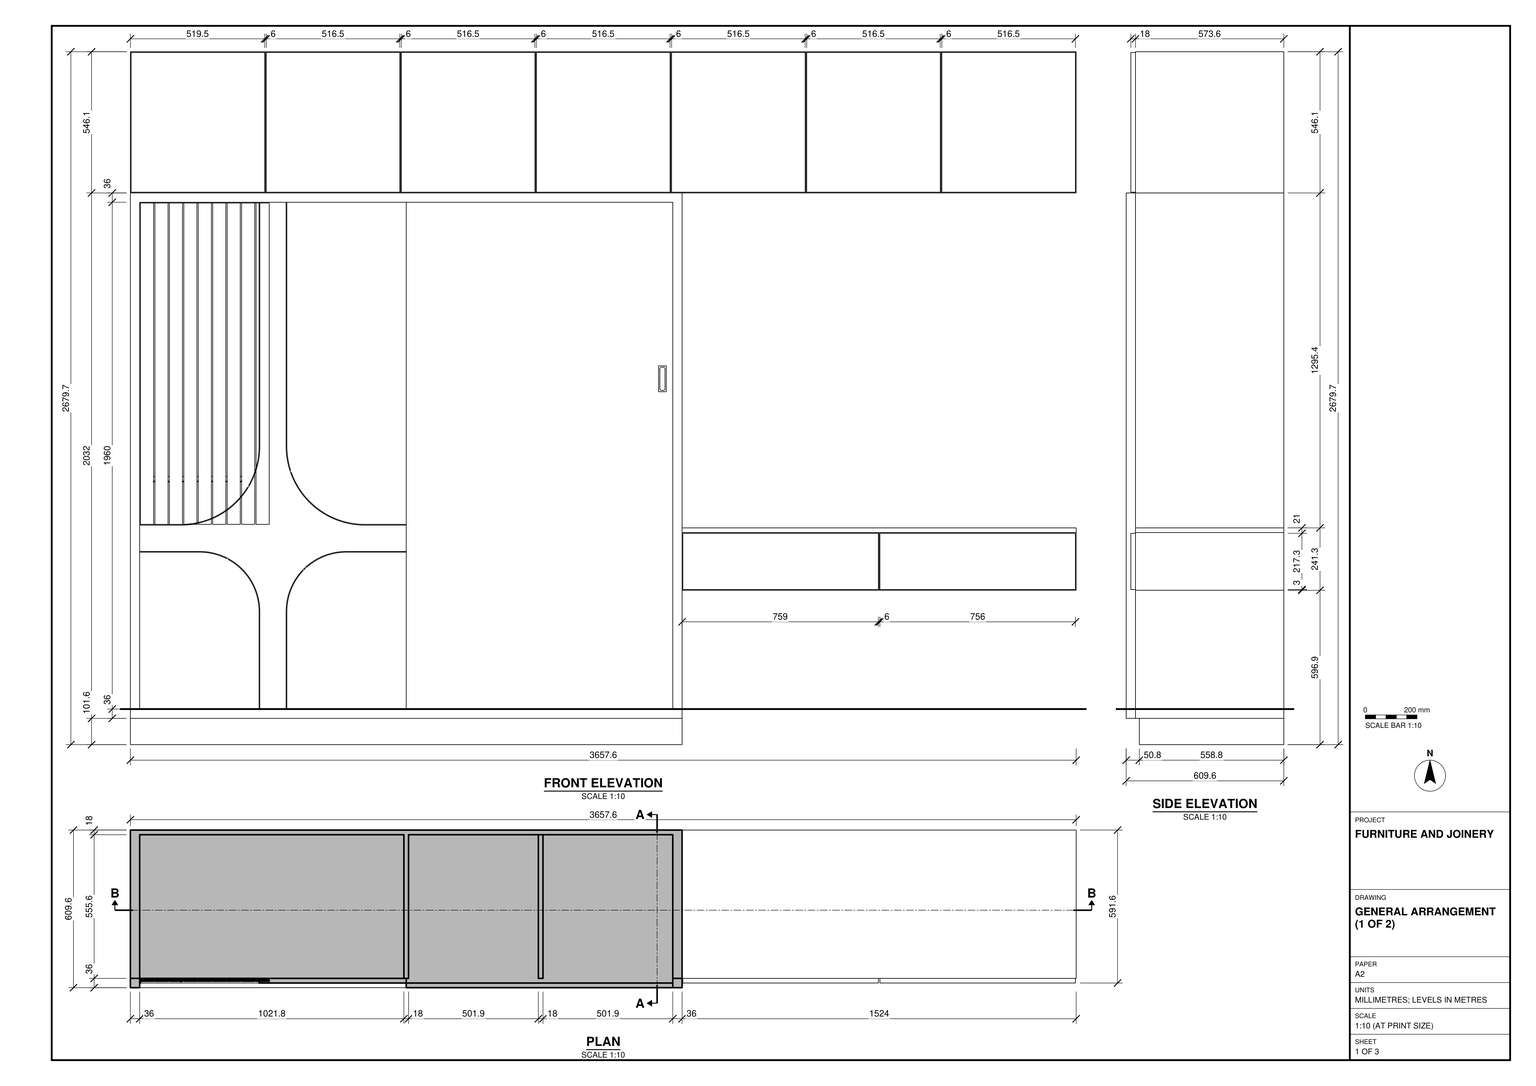
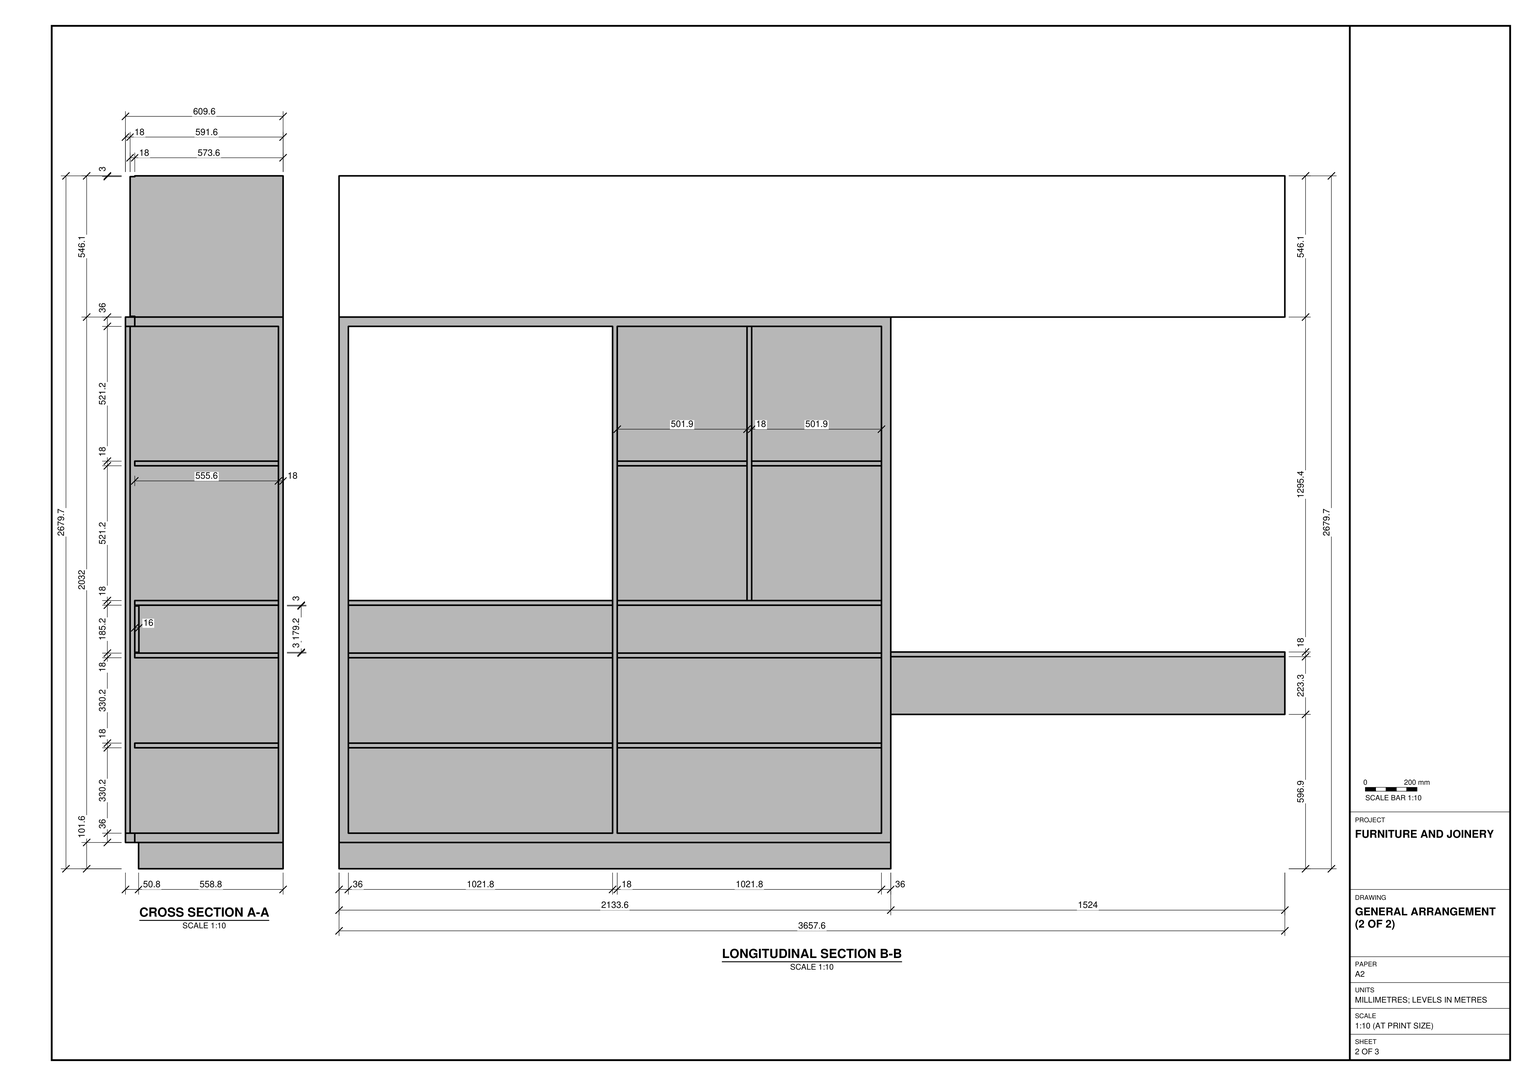
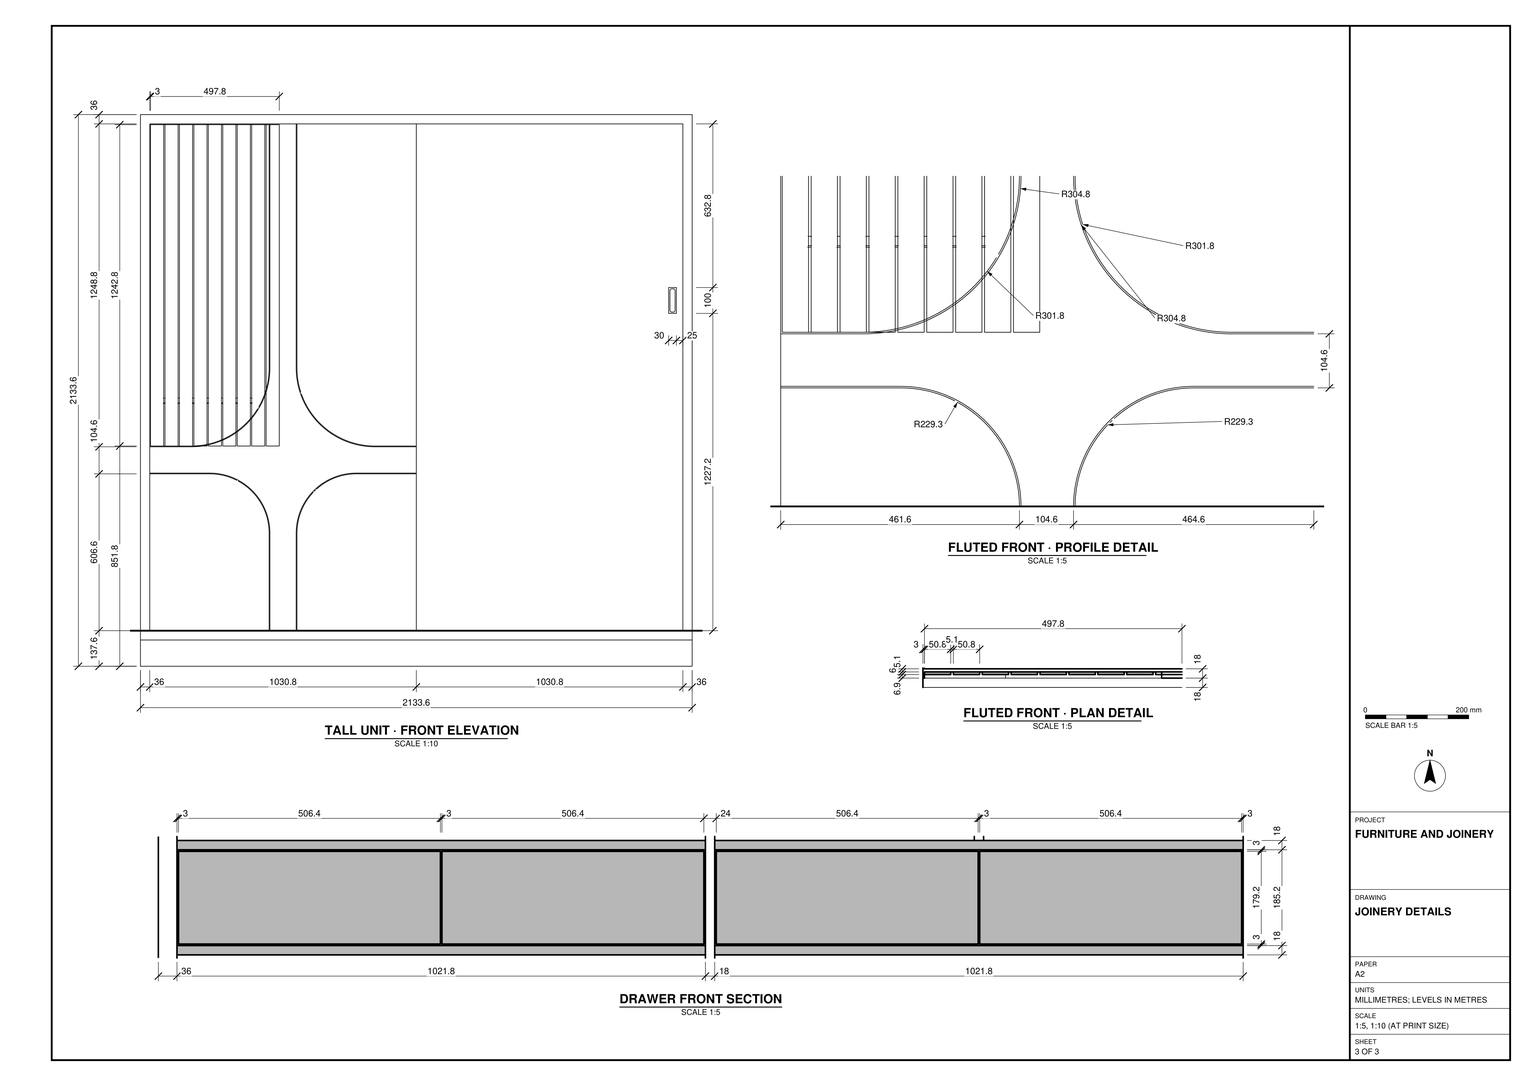
Build the storage joinery in SketchUp from task_files/diagram_01.pdf. Work in millimetres, with the underside of the plinth at ground level (±0.000, or 0 mm). Orient the front elevation along the X axis and the depth along the Y axis. The complete assembly is 3657.6 mm wide, 609.6 mm deep and 2679.7 mm high.

Run the seven overhead cupboard fronts across the full width. Below them, place the 2133.6 mm wide tall cabinet on the left and the 1524 mm wide floating drawer unit on the right. Keep the space above and below the floating unit open. Set back the tall cabinet’s plinth from its front face. Use the sections to model the cabinet interior behind the fronts, including the central partition, lower shelves, paired drawers in each bay and extra shelving in the upper right bay.

Use the third sheet for the two tall fronts. Form the vertical fluting in the upper left area of the patterned front and follow the drawn curves where the vertical and horizontal bands meet. Keep the adjoining front plain apart from its recessed rectangular pull. Model the panel thicknesses, front reveals and plinth setback shown in the sections rather than representing them with lines on a single face.

Keep the joinery units and their constituent parts separately editable as groups or components, and use components for repeated parts. Any decor or loose items may be suitable library components. Save one SketchUp model as output_files/storage_unit_with_upper_cupboards_and_floating_drawers.skp.

# SketchUp Ruby script. Lengths in millimetres.
U = 1.mm
M = Sketchup.active_model
def pt(a) = Geom::Point3d.new(a.map { |v| v * U })
def face(e, loops, mat)
  f = e.add_face(loops[0].map { |a| pt(a) })
  loops[1..].each { |l| e.add_face(l.map { |a| pt(a) }).erase! }
  f.material = f.back_material = mat if mat
  f
end
# faces: each face lists its corners as indices into pts; further lists are holes
def faces(e, pts, list, mat = nil) = list.each { |f| face(e, (f[0].is_a?(Array) ? f : [f]).map { |l| l.map { |i| pts[i] } }, mat) }
# xy, xz, yz: faces in a plane at the given z, y or x. An outline is a flat list of corners, or four numbers for a rectangle; further outlines are holes
def ring(l) = l.size == 4 ? [[l[0], l[1]], [l[2], l[1]], [l[2], l[3]], [l[0], l[3]]] : l.each_slice(2).to_a
def flat(e, list, mat, &to3) = list.each { |f| face(e, (f[0].is_a?(Array) ? f : [f]).map { |l| ring(l).map { |u, v| to3.(u, v) } }, mat) }
def xy(e, z, list, mat = nil) = flat(e, list, mat) { |x, y| [x, y, z] }
def xz(e, y, list, mat = nil) = flat(e, list, mat) { |x, z| [x, y, z] }
def yz(e, x, list, mat = nil) = flat(e, list, mat) { |y, z| [x, y, z] }
def lines(e, pts, list) = list.each { |a, b| e.add_line(pt(pts[a]), pt(pts[b])) }
# prism: a flat outline (further loops are holes) pulled along v
def prism(e, loops, v, mat = nil)
  f = face(e, loops, mat); d = Geom::Vector3d.new(v.map { |x| x * U })
  f.pushpull(f.normal.samedirection?(d) ? d.length : -d.length)
end
def box(e, o, s, mat = nil) = prism(e, [[o, [o[0] + s[0], o[1], o[2]], [o[0] + s[0], o[1] + s[1], o[2]], [o[0], o[1] + s[1], o[2]]]], [0, 0, s[2]], mat)
def at(x, y, z, deg = 0) = Geom::Transformation.translation(pt([x, y, z])) * Geom::Transformation.rotation(ORIGIN, Z_AXIS, deg.degrees)
def axes(o, x, y, z) = Geom::Transformation.new([*x, 0, *y, 0, *z, 0, *pt(o).to_a, 1])
def part(name) = M.definitions.add(name)
# library, detail: a bought-in or finely detailed component or shape, given as its bounding box
def library(name, o, s) = part(name).tap { |d| box(d.entities, o, s) }
def detail(e, o, s) = box(e.add_group.entities, o, s)
def put(e, d, t, mat = nil) = e.add_instance(d, t).tap { |i| i.material = mat if mat }
def group(e, t, mat = nil) = e.add_group.tap { |g| g.transformation = t; g.material = mat if mat }.entities
root = M.entities
c1 = part("Group\#2")
box(c1.entities,[-266.4,0,0],[1021.8,555.6,18])
c2 = part("Group\#7")
box(c2.entities,[0,0,0],[506.4,16,179.2])
c3 = part("Group\#8")
box(c3.entities,[0,0,0],[501.9,555.6,18])
xy(root,1037.2,[[1577.7,36,1595.7,591.6]])
xy(root,2097.6,[[1577.7,36,1595.7,591.6]])
xz(root,36,[[1577.7,1037.2,1595.7,2097.6]])
xz(root,591.6,[[1577.7,1037.2,1595.7,2097.6]])
yz(root,1577.7,[[36,1037.2,591.6,2097.6]])
yz(root,1595.7,[[36,1037.2,591.6,2097.6]])
p = [[1595.7,591.6,1567.4],[2097.6,591.6,1567.4]]
lines(root,p,[[0,1]])
g1 = group(root,at(0,0,101.6))
prism(g1,[[[0,36,0],[0,36,2032],[2133.6,36,2032],[2133.6,36,0]],[[2097.6,36,1996],[36,36,1996],[36,36,36],[2097.6,36,36]]],[0,-36,0])
g2 = group(root,at(0,0,0))
xy(g2,0,[[0,50.8,2133.6,609.6]])
xy(g2,101.6,[[0,36,2133.6,50.8],[0,50.8,2133.6,609.6]])
xy(g2,137.6,[[36,36,1057.8,591.6],[1075.8,36,2097.6,591.6]])
xy(g2,2097.6,[[36,36,1057.8,591.6],[1075.8,36,2097.6,591.6]])
xy(g2,2133.6,[[0,36,2133.6,609.6]])
xz(g2,36,[[[0,101.6,2133.6,2133.6],[36,137.6,2097.6,2097.6]],[1057.8,137.6,1075.8,2097.6]])
xz(g2,50.8,[[0,0,2133.6,101.6]])
xz(g2,591.6,[[36,137.6,1057.8,2097.6],[1075.8,137.6,2097.6,2097.6]])
xz(g2,609.6,[[0,0,2133.6,101.6],[0,101.6,2133.6,2133.6]])
yz(g2,0,[[50.8,0,609.6,101.6],[36,101.6,609.6,2133.6]])
yz(g2,36,[[36,137.6,591.6,2097.6]])
yz(g2,1057.8,[[36,137.6,591.6,2097.6]])
yz(g2,1075.8,[[36,137.6,591.6,2097.6]])
yz(g2,2097.6,[[36,137.6,591.6,2097.6]])
yz(g2,2133.6,[[50.8,0,609.6,101.6],[36,101.6,609.6,2133.6]])
g3 = group(root,at(36,18,137.6))
xy(g3,0,[[0,0,1030.8,18]])
xy(g3,714.2,[[3,0,159.8,12]])
xy(g3,1957,[[3,0,461.6,12]])
xy(g3,1960,[[0,0,1030.8,18]])
xz(g3,0,[[0,0,461.6,0,461.6,377.3,461.5,383.3,461.3,389.3,460.9,395.3,460.3,401.3,459.6,407.2,458.8,413.2,457.8,419.1,456.6,425,455.3,430.8,453.8,436.6,452.2,442.4,450.4,448.2,448.4,453.8,446.4,459.5,444.1,465,441.8,470.6,439.3,476,436.6,481.4,433.8,486.7,430.9,492,427.8,497.1,424.6,502.2,421.3,507.2,417.8,512.1,414.2,516.9,410.5,521.6,406.7,526.2,402.7,530.7,398.6,535.1,394.4,539.4,390.1,543.6,385.7,547.7,381.2,551.7,376.6,555.5,371.9,559.2,367.1,562.8,362.2,566.3,357.2,569.6,352.1,572.8,347,575.9,341.7,578.8,336.4,581.6,331,584.3,325.6,586.8,320,589.1,314.5,591.4,308.8,593.4,303.2,595.4,297.4,597.2,291.6,598.8,285.8,600.3,280,601.6,274.1,602.8,268.2,603.8,262.2,604.6,256.3,605.3,250.3,605.9,244.3,606.3,238.3,606.5,232.3,606.6,0,606.6],[461.6,0,464.6,0,464.6,377.3,464.5,383.4,464.3,389.5,463.9,395.5,463.3,401.6,462.6,407.6,461.7,413.6,460.7,419.6,459.5,425.6,458.2,431.5,456.7,437.4,455,443.3,453.2,449.1,451.3,454.8,449.2,460.5,446.9,466.2,444.5,471.8,442,477.3,439.3,482.8,436.4,488.1,433.5,493.5,430.4,498.7,427.1,503.8,423.7,508.9,420.2,513.8,416.6,518.7,412.8,523.5,408.9,528.2,404.9,532.7,400.8,537.2,396.6,541.6,392.2,545.8,387.7,549.9,383.2,553.9,378.5,557.8,373.7,561.6,368.8,565.2,363.9,568.7,358.8,572.1,353.7,575.4,348.5,578.5,343.1,581.4,337.8,584.3,332.3,587,326.8,589.5,321.2,591.9,315.5,594.2,309.8,596.3,304.1,598.2,298.3,600,292.4,601.7,286.5,603.2,280.6,604.5,274.6,605.7,268.6,606.7,262.6,607.6,256.6,608.3,250.5,608.9,244.5,609.3,238.4,609.5,232.3,609.6,0,609.6,0,606.6,232.3,606.6,238.3,606.5,244.3,606.3,250.3,605.9,256.3,605.3,262.2,604.6,268.2,603.8,274.1,602.8,280,601.6,285.8,600.3,291.6,598.8,297.4,597.2,303.2,595.4,308.8,593.4,314.5,591.4,320,589.1,325.6,586.8,331,584.3,336.4,581.6,341.7,578.8,347,575.9,352.1,572.8,357.2,569.6,362.2,566.3,367.1,562.8,371.9,559.2,376.6,555.5,381.2,551.7,385.7,547.7,390.1,543.6,394.4,539.4,398.6,535.1,402.7,530.7,406.7,526.2,410.5,521.6,414.2,516.9,417.8,512.1,421.3,507.2,424.6,502.2,427.8,497.1,430.9,492,433.8,486.7,436.6,481.4,439.3,476,441.8,470.6,444.1,465,446.4,459.5,448.4,453.8,450.4,448.2,452.2,442.4,453.8,436.6,455.3,430.8,456.6,425,457.8,419.1,458.8,413.2,459.6,407.2,460.3,401.3,460.9,395.3,461.3,389.3,461.5,383.3,461.6,377.3],[464.6,0,566.2,0,566.2,377.3,566.3,383.4,566.5,389.5,566.9,395.5,567.5,401.6,568.2,407.6,569.1,413.6,570.1,419.6,571.3,425.6,572.6,431.5,574.1,437.4,575.8,443.3,577.6,449.1,579.5,454.8,581.6,460.5,583.9,466.2,586.3,471.8,588.8,477.3,591.5,482.8,594.4,488.1,597.3,493.5,600.4,498.7,603.7,503.8,607.1,508.9,610.6,513.8,614.2,518.7,618,523.5,621.9,528.2,625.9,532.7,630,537.2,634.2,541.6,638.6,545.8,643.1,549.9,647.6,553.9,652.3,557.8,657.1,561.6,662,565.2,666.9,568.7,672,572.1,677.1,575.4,682.3,578.5,687.7,581.4,693,584.3,698.5,587,704,589.5,709.6,591.9,715.3,594.2,721,596.3,726.7,598.2,732.5,600,738.4,601.7,744.3,603.2,750.2,604.5,756.2,605.7,762.2,606.7,768.2,607.6,774.2,608.3,780.3,608.9,786.3,609.3,792.4,609.5,798.5,609.6,1030.8,609.6,1030.8,711.2,871,711.2,863,711.3,855,711.6,847.1,712.1,839.1,712.9,831.2,713.8,823.3,715,815.5,716.3,807.6,717.9,799.8,719.6,792.1,721.6,784.4,723.8,776.8,726.1,769.3,728.7,761.8,731.4,754.4,734.4,747,737.6,739.8,740.9,732.6,744.4,725.6,748.1,718.6,752,711.7,756.1,705,760.4,698.4,764.8,691.8,769.4,685.4,774.2,679.2,779.1,673,784.2,667,789.5,661.2,794.9,655.5,800.5,649.9,806.2,644.5,812,639.2,818,634.1,824.2,629.2,830.4,624.4,836.8,619.8,843.4,615.4,850,611.1,856.7,607,863.6,603.1,870.6,599.4,877.6,595.9,884.8,592.6,892,589.4,899.4,586.4,906.8,583.7,914.3,581.1,921.8,578.8,929.4,576.6,937.1,574.6,944.8,572.9,952.6,571.3,960.5,570,968.3,568.8,976.2,567.9,984.1,567.1,992.1,566.6,1000,566.3,1008,566.2,1016,566.2,1960,464.6,1960,464.6,1016,464.5,1008,464.2,1000,463.7,992.1,462.9,984.1,462,976.2,460.8,968.3,459.5,960.5,457.9,952.6,456.2,944.8,454.2,937.1,452,929.4,449.7,921.8,447.1,914.3,444.4,906.8,441.4,899.4,438.2,892,434.9,884.8,431.4,877.6,427.7,870.6,423.8,863.6,419.7,856.7,415.4,850,411,843.4,406.4,836.8,401.6,830.4,396.7,824.2,391.6,818,386.3,812,380.9,806.2,375.3,800.5,369.6,794.9,363.8,789.5,357.8,784.2,351.6,779.1,345.4,774.2,339,769.4,332.4,764.8,325.8,760.4,319.1,756.1,312.2,752,305.2,748.1,298.2,744.4,291,740.9,283.8,737.6,276.4,734.4,269,731.4,261.5,728.7,254,726.1,246.4,723.8,238.7,721.6,231,719.6,223.2,717.9,215.3,716.3,207.5,715,199.6,713.8,191.7,712.9,183.7,712.1,175.8,711.6,167.8,711.3,159.8,711.2,0,711.2,0,609.6,232.3,609.6,238.4,609.5,244.5,609.3,250.5,608.9,256.6,608.3,262.6,607.6,268.6,606.7,274.6,605.7,280.6,604.5,286.5,603.2,292.4,601.7,298.3,600,304.1,598.2,309.8,596.3,315.5,594.2,321.2,591.9,326.8,589.5,332.3,587,337.8,584.3,343.1,581.4,348.5,578.5,353.7,575.4,358.8,572.1,363.9,568.7,368.8,565.2,373.7,561.6,378.5,557.8,383.2,553.9,387.7,549.9,392.2,545.8,396.6,541.6,400.8,537.2,404.9,532.7,408.9,528.2,412.8,523.5,416.6,518.7,420.2,513.8,423.7,508.9,427.1,503.8,430.4,498.7,433.5,493.5,436.4,488.1,439.3,482.8,442,477.3,444.5,471.8,446.9,466.2,449.2,460.5,451.3,454.8,453.2,449.1,455,443.3,456.7,437.4,458.2,431.5,459.5,425.6,460.7,419.6,461.7,413.6,462.6,407.6,463.3,401.6,463.9,395.5,464.3,389.5,464.5,383.4,464.6,377.3],[566.2,0,569.2,0,569.2,377.3,569.3,383.3,569.5,389.3,569.9,395.3,570.5,401.3,571.2,407.2,572,413.2,573,419.1,574.2,425,575.5,430.8,577,436.6,578.6,442.4,580.4,448.2,582.4,453.8,584.4,459.5,586.7,465,589,470.6,591.5,476,594.2,481.4,597,486.7,599.9,492,603,497.1,606.2,502.2,609.5,507.2,613,512.1,616.6,516.9,620.3,521.6,624.1,526.2,628.1,530.7,632.2,535.1,636.4,539.4,640.7,543.6,645.1,547.7,649.6,551.7,654.2,555.5,658.9,559.2,663.7,562.8,668.6,566.3,673.6,569.6,678.7,572.8,683.8,575.9,689.1,578.8,694.4,581.6,699.8,584.3,705.2,586.8,710.8,589.1,716.3,591.4,722,593.4,727.6,595.4,733.4,597.2,739.2,598.8,745,600.3,750.8,601.6,756.7,602.8,762.6,603.8,768.6,604.6,774.5,605.3,780.5,605.9,786.5,606.3,792.5,606.5,798.5,606.6,1030.8,606.6,1030.8,609.6,798.5,609.6,792.4,609.5,786.3,609.3,780.3,608.9,774.2,608.3,768.2,607.6,762.2,606.7,756.2,605.7,750.2,604.5,744.3,603.2,738.4,601.7,732.5,600,726.7,598.2,721,596.3,715.3,594.2,709.6,591.9,704,589.5,698.5,587,693,584.3,687.7,581.4,682.3,578.5,677.1,575.4,672,572.1,666.9,568.7,662,565.2,657.1,561.6,652.3,557.8,647.6,553.9,643.1,549.9,638.6,545.8,634.2,541.6,630,537.2,625.9,532.7,621.9,528.2,618,523.5,614.2,518.7,610.6,513.8,607.1,508.9,603.7,503.8,600.4,498.7,597.3,493.5,594.4,488.1,591.5,482.8,588.8,477.3,586.3,471.8,583.9,466.2,581.6,460.5,579.5,454.8,577.6,449.1,575.8,443.3,574.1,437.4,572.6,431.5,571.3,425.6,570.1,419.6,569.1,413.6,568.2,407.6,567.5,401.6,566.9,395.5,566.5,389.5,566.3,383.4,566.2,377.3],[569.2,0,1030.8,0,1030.8,606.6,798.5,606.6,792.5,606.5,786.5,606.3,780.5,605.9,774.5,605.3,768.6,604.6,762.6,603.8,756.7,602.8,750.8,601.6,745,600.3,739.2,598.8,733.4,597.2,727.6,595.4,722,593.4,716.3,591.4,710.8,589.1,705.2,586.8,699.8,584.3,694.4,581.6,689.1,578.8,683.8,575.9,678.7,572.8,673.6,569.6,668.6,566.3,663.7,562.8,658.9,559.2,654.2,555.5,649.6,551.7,645.1,547.7,640.7,543.6,636.4,539.4,632.2,535.1,628.1,530.7,624.1,526.2,620.3,521.6,616.6,516.9,613,512.1,609.5,507.2,606.2,502.2,603,497.1,599.9,492,597,486.7,594.2,481.4,591.5,476,589,470.6,586.7,465,584.4,459.5,582.4,453.8,580.4,448.2,578.6,442.4,577,436.6,575.5,430.8,574.2,425,573,419.1,572,413.2,571.2,407.2,570.5,401.3,569.9,395.3,569.5,389.3,569.3,383.3,569.2,377.3],
  [[0,711.2,159.8,711.2,167.8,711.3,175.8,711.6,183.7,712.1,191.7,712.9,199.6,713.8,207.5,715,215.3,716.3,223.2,717.9,231,719.6,238.7,721.6,246.4,723.8,254,726.1,261.5,728.7,269,731.4,276.4,734.4,283.8,737.6,291,740.9,298.2,744.4,305.2,748.1,312.2,752,319.1,756.1,325.8,760.4,332.4,764.8,339,769.4,345.4,774.2,351.6,779.1,357.8,784.2,363.8,789.5,369.6,794.9,375.3,800.5,380.9,806.2,386.3,812,391.6,818,396.7,824.2,401.6,830.4,406.4,836.8,411,843.4,415.4,850,419.7,856.7,423.8,863.6,427.7,870.6,431.4,877.6,434.9,884.8,438.2,892,441.4,899.4,444.4,906.8,447.1,914.3,449.7,921.8,452,929.4,454.2,937.1,456.2,944.8,457.9,952.6,459.5,960.5,460.8,968.3,462,976.2,462.9,984.1,463.7,992.1,464.2,1000,464.5,1008,464.6,1016,464.6,1960,0,1960],[3,714.2,3,1957,461.6,1957,461.6,1016,461.5,1008.1,461.2,1000.2,460.7,992.3,459.9,984.5,459,976.6,457.9,968.8,456.5,961,455,953.3,453.3,945.5,451.3,937.9,449.2,930.3,446.8,922.7,444.3,915.3,441.6,907.8,438.6,900.5,435.5,893.2,432.2,886.1,428.7,879,425,872,421.2,865.1,417.1,858.3,412.9,851.6,408.5,845.1,404,838.6,399.2,832.3,394.3,826.1,389.3,820,384.1,814.1,378.7,808.3,373.2,802.6,367.5,797.1,361.7,791.7,355.8,786.5,349.7,781.5,343.5,776.6,337.2,771.8,330.7,767.3,324.2,762.9,317.5,758.7,310.7,754.6,303.8,750.8,296.8,747.1,289.7,743.6,282.6,740.3,275.3,737.2,268,734.2,260.5,731.5,253.1,729,245.5,726.6,237.9,724.5,230.3,722.5,222.5,720.8,214.8,719.3,207,717.9,199.2,716.8,191.3,715.9,183.5,715.1,175.6,714.6,167.7,714.3,159.8,714.2]],[871,711.2,1030.8,711.2,1030.8,714.2,871,714.2,863.1,714.3,855.2,714.6,847.3,715.1,839.5,715.9,831.6,716.8,823.8,717.9,816,719.3,808.3,720.8,800.5,722.5,792.9,724.5,785.3,726.6,777.7,729,770.3,731.5,762.8,734.2,755.5,737.2,748.2,740.3,741.1,743.6,734,747.1,727,750.8,720.1,754.6,713.3,758.7,706.6,762.9,700.1,767.3,693.6,771.8,687.3,776.6,681.1,781.5,675,786.5,669.1,791.7,663.3,797.1,657.6,802.6,652.1,808.3,646.7,814.1,641.5,820,636.5,826.1,631.6,832.3,626.8,838.6,622.3,845.1,617.9,851.6,613.7,858.3,609.6,865.1,605.8,872,602.1,879,598.6,886.1,595.3,893.2,592.2,900.5,589.2,907.8,586.5,915.3,584,922.7,581.6,930.3,579.5,937.9,577.5,945.5,575.8,953.3,574.3,961,572.9,968.8,571.8,976.6,570.9,984.5,570.1,992.3,569.6,1000.2,569.3,1008.1,569.2,1016,569.2,1960,566.2,1960,566.2,1016,566.3,1008,566.6,1000,567.1,992.1,567.9,984.1,568.8,976.2,570,968.3,571.3,960.5,572.9,952.6,574.6,944.8,576.6,937.1,578.8,929.4,581.1,921.8,583.7,914.3,586.4,906.8,589.4,899.4,592.6,892,595.9,884.8,599.4,877.6,603.1,870.6,607,863.6,611.1,856.7,615.4,850,619.8,843.4,624.4,836.8,629.2,830.4,634.1,824.2,639.2,818,644.5,812,649.9,806.2,655.5,800.5,661.2,794.9,667,789.5,673,784.2,679.2,779.1,685.4,774.2,691.8,769.4,698.4,764.8,705,760.4,711.7,756.1,718.6,752,725.6,748.1,732.6,744.4,739.8,740.9,747,737.6,754.4,734.4,761.8,731.4,769.3,728.7,776.8,726.1,784.4,723.8,792.1,721.6,799.8,719.6,807.6,717.9,815.5,716.3,823.3,715,831.2,713.8,839.1,712.9,847.1,712.1,855,711.6,863,711.3],[871,714.2,1030.8,714.2,1030.8,1960,569.2,1960,569.2,1016,569.3,1008.1,569.6,1000.2,570.1,992.3,570.9,984.5,571.8,976.6,572.9,968.8,574.3,961,575.8,953.3,577.5,945.5,579.5,937.9,581.6,930.3,584,922.7,586.5,915.3,589.2,907.8,592.2,900.5,595.3,893.2,598.6,886.1,602.1,879,605.8,872,609.6,865.1,613.7,858.3,617.9,851.6,622.3,845.1,626.8,838.6,631.6,832.3,636.5,826.1,641.5,820,646.7,814.1,652.1,808.3,657.6,802.6,663.3,797.1,669.1,791.7,675,786.5,681.1,781.5,687.3,776.6,693.6,771.8,700.1,767.3,706.6,762.9,713.3,758.7,720.1,754.6,727,750.8,734,747.1,741.1,743.6,748.2,740.3,755.5,737.2,762.8,734.2,770.3,731.5,777.7,729,785.3,726.6,792.9,724.5,800.5,722.5,808.3,720.8,816,719.3,823.8,717.9,831.6,716.8,839.5,715.9,847.3,715.1,855.2,714.6,863.1,714.3]])
xz(g3,12,[[3,714.2,159.8,714.2,167.7,714.3,175.6,714.6,183.5,715.1,191.3,715.9,199.2,716.8,207,717.9,214.8,719.3,222.5,720.8,230.3,722.5,237.9,724.5,245.5,726.6,253.1,729,260.5,731.5,268,734.2,275.3,737.2,282.6,740.3,289.7,743.6,296.8,747.1,303.8,750.8,310.7,754.6,317.5,758.7,324.2,762.9,330.7,767.3,337.2,771.8,343.5,776.6,349.7,781.5,355.8,786.5,361.7,791.7,367.5,797.1,373.2,802.6,378.7,808.3,384.1,814.1,389.3,820,394.3,826.1,399.2,832.3,404,838.6,408.5,845.1,412.9,851.6,417.1,858.3,421.2,865.1,425,872,428.7,879,432.2,886.1,435.5,893.2,438.6,900.5,441.6,907.8,444.3,915.3,446.8,922.7,449.2,930.3,451.3,937.9,453.3,945.5,455,953.3,456.5,961,457.9,968.8,459,976.6,459.9,984.5,460.7,992.3,461.2,1000.2,461.5,1008.1,461.6,1016,461.6,1957,3,1957]])
xz(g3,18,[[0,0,1030.8,1960]])
yz(g3,0,[[0,0,18,1960]])
yz(g3,3,[[0,714.2,12,1957]])
yz(g3,461.6,[[0,1016,12,1957]])
yz(g3,1030.8,[[0,0,18,1960]])
p = [[159.8,0,714.2],[167.7,0,714.3],[167.7,12,714.3],[159.8,12,714.2],[175.6,0,714.6],[175.6,12,714.6],
  [183.5,0,715.1],[183.5,12,715.1],[191.3,0,715.9],[191.3,12,715.9],[199.2,0,716.8],[199.2,12,716.8],
  [207,0,717.9],[207,12,717.9],[214.8,0,719.3],[214.8,12,719.3],[222.5,0,720.8],[222.5,12,720.8],
  [230.3,0,722.5],[230.3,12,722.5],[237.9,0,724.5],[237.9,12,724.5],[245.5,0,726.6],[245.5,12,726.6],
  [253.1,0,729],[253.1,12,729],[260.5,0,731.5],[260.5,12,731.5],[268,0,734.2],[268,12,734.2],
  [275.3,0,737.2],[275.3,12,737.2],[282.6,0,740.3],[282.6,12,740.3],[289.7,0,743.6],[289.7,12,743.6],
  [296.8,0,747.1],[296.8,12,747.1],[303.8,0,750.8],[303.8,12,750.8],[310.7,0,754.6],[310.7,12,754.6],
  [317.5,0,758.7],[317.5,12,758.7],[324.2,0,762.9],[324.2,12,762.9],[330.7,0,767.3],[330.7,12,767.3],
  [337.2,0,771.8],[337.2,12,771.8],[343.5,0,776.6],[343.5,12,776.6],[349.7,0,781.5],[349.7,12,781.5],
  [355.8,0,786.5],[355.8,12,786.5],[361.7,0,791.7],[361.7,12,791.7],[367.5,0,797.1],[367.5,12,797.1],
  [373.2,0,802.6],[373.2,12,802.6],[378.7,0,808.3],[378.7,12,808.3],[384.1,0,814.1],[384.1,12,814.1],
  [389.3,0,820],[389.3,12,820],[394.3,0,826.1],[394.3,12,826.1],[399.2,0,832.3],[399.2,12,832.3],
  [404,0,838.6],[404,12,838.6],[408.5,0,845.1],[408.5,12,845.1],[412.9,0,851.6],[412.9,12,851.6],
  [417.1,0,858.3],[417.1,12,858.3],[421.2,0,865.1],[421.2,12,865.1],[425,0,872],[425,12,872],
  [428.7,0,879],[428.7,12,879],[432.2,0,886.1],[432.2,12,886.1],[435.5,0,893.2],[435.5,12,893.2],
  [438.6,0,900.5],[438.6,12,900.5],[441.6,0,907.8],[441.6,12,907.8],[444.3,0,915.3],[444.3,12,915.3],
  [446.8,0,922.7],[446.8,12,922.7],[449.2,0,930.3],[449.2,12,930.3],[451.3,0,937.9],[451.3,12,937.9],
  [453.3,0,945.5],[453.3,12,945.5],[455,0,953.3],[455,12,953.3],[456.5,0,961],[456.5,12,961],
  [457.9,0,968.8],[457.9,12,968.8],[459,0,976.6],[459,12,976.6],[459.9,0,984.5],[459.9,12,984.5],
  [460.7,0,992.3],[460.7,12,992.3],[461.2,0,1000.2],[461.2,12,1000.2],[461.5,0,1008.1],[461.5,12,1008.1],
  [461.6,0,1016],[461.6,12,1016]]
faces(g3,p,[[0,1,2,3],[1,4,5,2],[4,6,7,5],[6,8,9,7],[8,10,11,9],[10,12,13,11],[12,14,15,13],[14,16,17,15],
  [16,18,19,17],[18,20,21,19],[20,22,23,21],[22,24,25,23],[24,26,27,25],[26,28,29,27],[28,30,31,29],[30,32,33,31],
  [32,34,35,33],[34,36,37,35],[36,38,39,37],[38,40,41,39],[40,42,43,41],[42,44,45,43],[44,46,47,45],[46,48,49,47],
  [48,50,51,49],[50,52,53,51],[52,54,55,53],[54,56,57,55],[56,58,59,57],[58,60,61,59],[60,62,63,61],[62,64,65,63],
  [64,66,67,65],[66,68,69,67],[68,70,71,69],[70,72,73,71],[72,74,75,73],[74,76,77,75],[76,78,79,77],[78,80,81,79],
  [80,82,83,81],[82,84,85,83],[84,86,87,85],[86,88,89,87],[88,90,91,89],[90,92,93,91],[92,94,95,93],[94,96,97,95],
  [96,98,99,97],[98,100,101,99],[100,102,103,101],[102,104,105,103],[104,106,107,105],[106,108,109,107],[108,110,111,109],[110,112,113,111],
  [112,114,115,113],[114,116,117,115],[116,118,119,117],[118,120,121,119]])
put(root,c1,at(302.4,36,816))
put(root,c1,at(302.4,36,467.8))
g4 = group(root,at(2097.6,0,137.6))
xy(g4,0,[[-1030.8,0,0,18]])
xy(g4,1960,[[-1030.8,0,0,18]])
xz(g4,0,[[[-1030.8,0,0,1960],[-55,1227.2,-25,1327.2]]])
xz(g4,18,[[-1030.8,0,0,1960]])
yz(g4,-1030.8,[[0,0,18,1960]])
yz(g4,0,[[0,0,18,1960]])
p = [[-35.2,0,1232.5],[-36.1,0,1232.3],[-49.8,0,1237.4],[-49.9,0,1238.3],[-33.5,0,1321.3],[-32.7,0,1320.8],
  [-47.9,0,1320.2],[-47.3,0,1320.8],[-32.7,0,1233.7],[-33.5,0,1233.2],[-30.2,0,1317],[-30.1,0,1316.1],
  [-30.9,0,1318.7],[-30.5,0,1317.9],[-43.9,0,1232.3],[-44.8,0,1232.5],[-34.3,0,1321.7],[-31.4,0,1319.5],
  [-30,0,1315.2],[-48.6,0,1319.5],[-47.9,0,1234.3],[-48.6,0,1235],[-30.5,0,1236.5],[-30.9,0,1235.7],
  [-49.1,0,1235.7],[-30.2,0,1237.4],[-34.3,0,1232.7],[-37,0,1322.2],[-36.1,0,1322.2],[-32.1,0,1320.2],
  [-49.5,0,1236.5],[-49.5,0,1317.9],[-49.1,0,1318.7],[-37,0,1232.2],[-49.9,0,1316.1],[-49.8,0,1317],
  [-46.5,0,1321.3],[-43,0,1232.2],[-45.7,0,1321.7],[-44.8,0,1322],[-32.1,0,1234.3],[-31.4,0,1235],
  [-30,0,1239.2],[-43.9,0,1322.2],[-50,0,1239.2],[-35.2,0,1322],[-43,0,1322.2],[-45.7,0,1232.7],
  [-46.5,0,1233.2],[-50,0,1315.2],[-47.3,0,1233.7],[-30.1,0,1238.3],[-50,0,1316.2]]
lines(g4,p,[[0,1],[2,3],[4,5],[6,7],[8,9],[10,11],[12,13],[14,15],[16,4],[17,12],[11,18],[19,6],
  [20,21],[22,23],[21,24],[25,22],[26,0],[27,28],[5,29],[24,30],[31,32],[1,33],[34,35],[7,36],
  [9,26],[37,14],[29,17],[32,19],[38,39],[40,8],[23,41],[18,42],[36,38],[39,43],[3,44],[45,16],
  [46,27],[28,45],[13,10],[30,2],[43,46],[47,48],[49,34],[48,50],[51,25],[33,37],[42,51],[41,40],
  [44,49],[50,20],[15,47],[35,31],[49,52]])
put(root,c1,at(302.4,36,1019.2))
g5 = group(root,at(1586.7,591.6,1037.2))
p = [[-9,0,0],[-9,0,1060.4],[9,0,0],[9,0,1060.4]]
lines(g5,p,[[0,1],[2,3]])
g6 = group(root,at(36,52,834))
xz(g6,0,[[[0,0,510.9,185.2],[3,3,509.4,182.2]],[[510.9,0,1021.8,185.2],[512.4,3,1018.8,182.2]]])
put(g6,c2,at(3,-16,3))
put(g6,c2,at(512.4,-16,3))
put(g6,c2,at(1552.2,-16,3))
put(g6,c2,at(1042.8,-16,3))
put(root,c1,at(1342.2,36,1019.2))
g7 = group(root,at(1075.8,52,834))
xz(g7,0,[[[0,0,510.9,185.2],[3,3,509.4,182.2]],[[510.9,0,1021.8,185.2],[512.4,3,1018.8,182.2]]])
put(root,c3,at(1595.7,36,1558.4))
g8 = group(root,at(0,36,2133.6))
xy(g8,0,[[0,0,3657.6,573.6]])
xy(g8,3,[[3,-18,519.5,0],[525.5,-18,1042,0],[1048,-18,1564.5,0],[1570.5,-18,2087.1,0],[2093.1,-18,2609.6,0],
  [2615.6,-18,3132.1,0],[3138.1,-18,3654.6,0]])
xy(g8,543.1,[[3,-18,519.5,0],[525.5,-18,1042,0],[1048,-18,1564.5,0],[1570.5,-18,2087.1,0],[2093.1,-18,2609.6,0],
  [2615.6,-18,3132.1,0],[3138.1,-18,3654.6,0]])
xy(g8,546.1,[[0,0,3657.6,573.6]])
xz(g8,-18,[[3,3,519.5,543.1],[525.5,3,1042,543.1],[1048,3,1564.5,543.1],[1570.5,3,2087.1,543.1],[2093.1,3,2609.6,543.1],
  [2615.6,3,3132.1,543.1],[3138.1,3,3654.6,543.1]])
xz(g8,0,[[[0,0,522.5,546.1],[3,3,519.5,543.1]],[[522.5,0,1045,546.1],[525.5,3,1042,543.1]],[[1045,0,1567.5,546.1],[1048,3,1564.5,543.1]],[[1567.5,0,2090.1,546.1],[1570.5,3,2087.1,543.1]],[[2090.1,0,2612.6,546.1],[2093.1,3,2609.6,543.1]],
  [[2612.6,0,3135.1,546.1],[2615.6,3,3132.1,543.1]],[[3135.1,0,3657.6,546.1],[3138.1,3,3654.6,543.1]]])
xz(g8,573.6,[[0,0,3657.6,546.1]])
yz(g8,0,[[0,0,573.6,546.1]])
yz(g8,3,[[-18,3,0,543.1]])
yz(g8,519.5,[[-18,3,0,543.1]])
yz(g8,525.5,[[-18,3,0,543.1]])
yz(g8,1042,[[-18,3,0,543.1]])
yz(g8,1048,[[-18,3,0,543.1]])
yz(g8,1564.5,[[-18,3,0,543.1]])
yz(g8,1570.5,[[-18,3,0,543.1]])
yz(g8,2087.1,[[-18,3,0,543.1]])
yz(g8,2093.1,[[-18,3,0,543.1]])
yz(g8,2609.6,[[-18,3,0,543.1]])
yz(g8,2615.6,[[-18,3,0,543.1]])
yz(g8,3132.1,[[-18,3,0,543.1]])
yz(g8,3138.1,[[-18,3,0,543.1]])
yz(g8,3654.6,[[-18,3,0,543.1]])
yz(g8,3657.6,[[0,0,573.6,546.1]])
put(root,c3,at(1075.8,36,1558.4))
g9 = group(root,at(2133.6,0,596.9))
xy(g9,0,[[0,36,1524,609.6]])
xy(g9,3,[[3,18,759,36],[765,18,1521,36]])
xy(g9,220.3,[[3,18,759,36],[765,18,1521,36]])
xy(g9,223.3,[[0,36,1524,609.6]])
xy(g9,241.3,[[0,36,1524,609.6]])
xz(g9,18,[[3,3,759,220.3],[765,3,1521,220.3]])
xz(g9,36,[[[0,0,762,223.3],[3,3,759,220.3]],[[762,0,1524,223.3],[765,3,1521,220.3]],[0,223.3,1524,241.3]])
xz(g9,609.6,[[0,0,1524,223.3],[0,223.3,1524,241.3]])
yz(g9,0,[[36,0,609.6,223.3],[36,223.3,609.6,241.3]])
yz(g9,3,[[18,3,36,220.3]])
yz(g9,759,[[18,3,36,220.3]])
yz(g9,765,[[18,3,36,220.3]])
yz(g9,1521,[[18,3,36,220.3]])
yz(g9,1524,[[36,0,609.6,223.3],[36,223.3,609.6,241.3]])
g10 = group(root,at(39,30,851.8))
box(g10,[0,-5.1,0],[50.8,5.1,1242.8])
box(g10,[55.9,-5.1,0],[50.8,5.1,1242.8])
box(g10,[111.8,-5.1,0],[50.8,5.1,1242.8])
box(g10,[167.6,-5.1,0],[50.8,5.1,1242.8])
box(g10,[223.5,-5.1,0],[50.8,5.1,1242.8])
box(g10,[279.4,-5.1,0],[50.8,5.1,1242.8])
box(g10,[335.3,-5.1,0],[50.8,5.1,1242.8])
box(g10,[391.2,-5.1,0],[50.8,5.1,1242.8])
box(g10,[447,-5.1,0],[50.8,5.1,1242.8])
put(root,c1,at(1342.2,36,816))
put(root,c1,at(1342.2,36,467.8))
